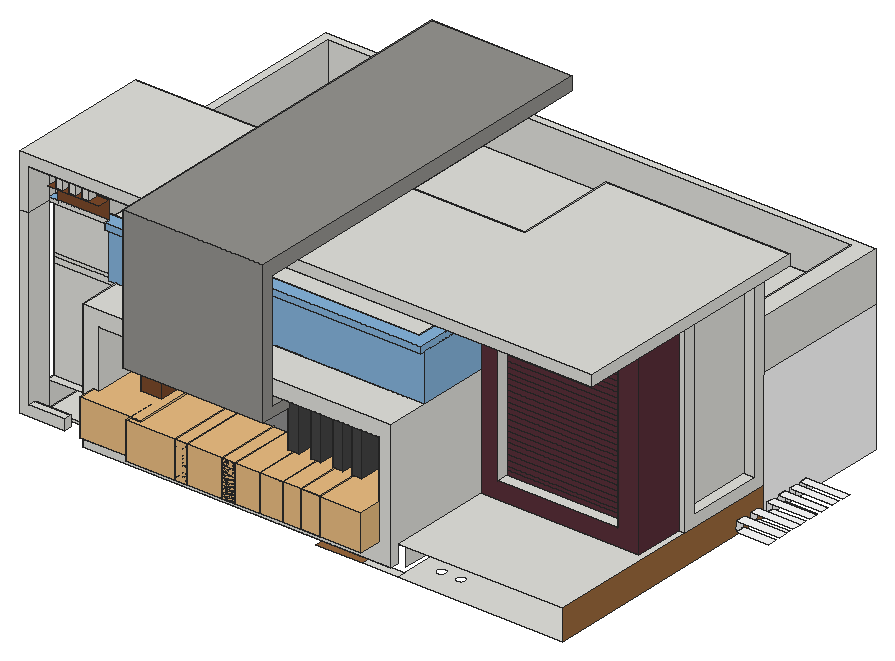
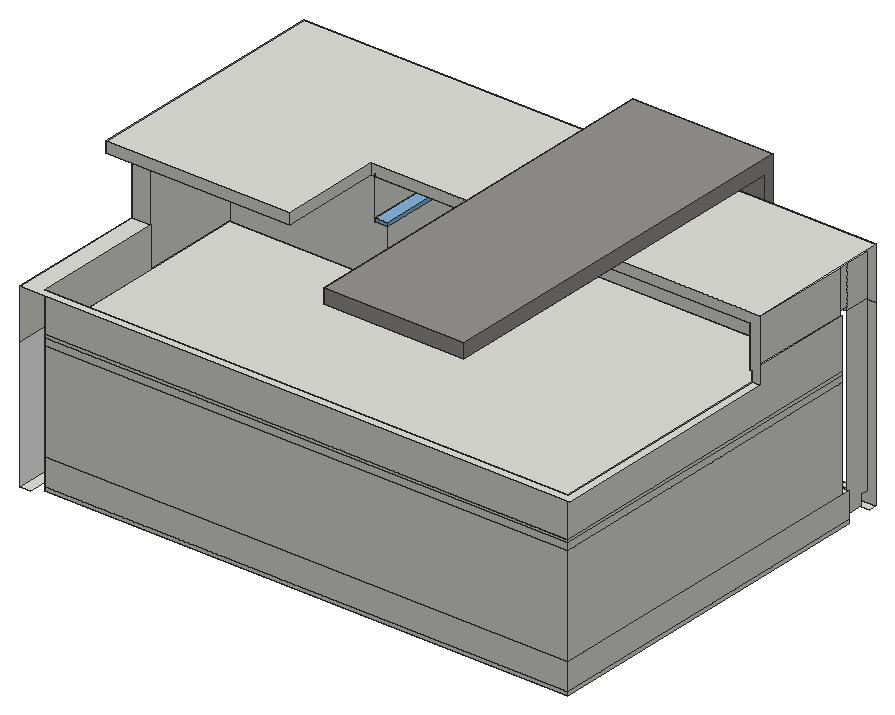
# SketchUp Ruby script. Lengths in inches.
U = 1.inch
M = Sketchup.active_model
def pt(a) = Geom::Point3d.new(a.map { |v| v * U })
def face(e, loops, mat)
  f = e.add_face(loops[0].map { |a| pt(a) })
  loops[1..].each { |l| e.add_face(l.map { |a| pt(a) }).erase! }
  f.material = f.back_material = mat if mat
  f
end
# faces: each face lists its corners as indices into pts; further lists are holes
def faces(e, pts, list, mat = nil) = list.each { |f| face(e, (f[0].is_a?(Array) ? f : [f]).map { |l| l.map { |i| pts[i] } }, mat) }
# xy, xz, yz: faces in a plane at the given z, y or x. An outline is a flat list of corners, or four numbers for a rectangle; further outlines are holes
def ring(l) = l.size == 4 ? [[l[0], l[1]], [l[2], l[1]], [l[2], l[3]], [l[0], l[3]]] : l.each_slice(2).to_a
def flat(e, list, mat, &to3) = list.each { |f| face(e, (f[0].is_a?(Array) ? f : [f]).map { |l| ring(l).map { |u, v| to3.(u, v) } }, mat) }
def xy(e, z, list, mat = nil) = flat(e, list, mat) { |x, y| [x, y, z] }
def xz(e, y, list, mat = nil) = flat(e, list, mat) { |x, z| [x, y, z] }
def yz(e, x, list, mat = nil) = flat(e, list, mat) { |y, z| [x, y, z] }
def lines(e, pts, list) = list.each { |a, b| e.add_line(pt(pts[a]), pt(pts[b])) }
# prism: a flat outline (further loops are holes) pulled along v
def prism(e, loops, v, mat = nil)
  f = face(e, loops, mat); d = Geom::Vector3d.new(v.map { |x| x * U })
  f.pushpull(f.normal.samedirection?(d) ? d.length : -d.length)
end
def box(e, o, s, mat = nil) = prism(e, [[o, [o[0] + s[0], o[1], o[2]], [o[0] + s[0], o[1] + s[1], o[2]], [o[0], o[1] + s[1], o[2]]]], [0, 0, s[2]], mat)
def at(x, y, z, deg = 0) = Geom::Transformation.translation(pt([x, y, z])) * Geom::Transformation.rotation(ORIGIN, Z_AXIS, deg.degrees)
def axes(o, x, y, z) = Geom::Transformation.new([*x, 0, *y, 0, *z, 0, *pt(o).to_a, 1])
def part(name) = M.definitions.add(name)
# library, detail: a bought-in or finely detailed component or shape, given as its bounding box
def library(name, o, s) = part(name).tap { |d| box(d.entities, o, s) }
def detail(e, o, s) = box(e.add_group.entities, o, s)
def put(e, d, t, mat = nil) = e.add_instance(d, t).tap { |i| i.material = mat if mat }
def group(e, t, mat = nil) = e.add_group.tap { |g| g.transformation = t; g.material = mat if mat }.entities
root = M.entities
M.materials.add("[Color I06]").color = [134, 181, 221]
M.materials.add("[Color L16]").color = [89, 47, 58]
M.materials.add("[Color M00]").color = [255, 255, 255]
M.materials.add("[Color M02]").color = [198, 198, 198]
M.materials.add("[Color M03]").color = [186, 170, 170]
M.materials.add("[Color M04]").color = [142, 142, 142]
M.materials.add("[Color M08]").color = [30, 30, 30]
M.materials.add("[Concrete Aggregate Smoke]").color = [154, 150, 148]
M.materials.add("[Granite Dark Gray]").color = [69, 68, 68]
M.materials.add("[Granite Light Gray]").color = [149, 148, 144]
M.materials.add("[Wood Floor Dark]").color = [123, 73, 42]
M.materials.add("[Wood Floor]").color = [155, 105, 61]
c1 = library("SimLab\#1",[-34.39,-41.14,-1.55],[72.52,77.18,43.59])
xy(root,129,[[514.48,231,557.08,241.25],[[557.08,231,754.5,408.375],[582.5,258.46,583.98,258.6,585.375,259.11,586.59,259.96,587.54,261.1,588.16,262.45,588.42,263.91,588.28,265.39,587.77,266.78,586.92,268,585.78,268.95,584.43,269.57,582.97,269.83,581.49,269.69,580.09,269.18,578.88,268.33,577.93,267.1875,577.3,265.84,577.05,264.38,577.18,262.9,577.7,261.51,578.55,260.29,579.69,259.34,581.04,258.72],[605.875,258.46,607.35,258.6,608.75,259.11,609.96,259.96,610.91,261.1,611.54,262.45,611.79,263.91,611.66,265.39,611.15,266.78,610.29,268,609.15,268.95,607.8,269.57,606.34,269.83,604.86,269.69,603.47,269.18,602.25,268.33,601.3,267.1875,600.68,265.84,600.43,264.38,600.56,262.9,601.07,261.51,601.93,260.29,603.07,259.34,604.41,258.72]],[103.75,271.1875,103.75,691.8125,732.0625,691.8125,732.0625,414.375,551.08,414.375,551.08,281.3125,105.9,271.1875],[741.0625,408.375,741.0625,700.8125,754.5625,700.8125,754.5625,533.07,754.5,533.07,754.5,408.375]])
xy(root,129,[[469.85,240.4375,471.69,241.25]],"[Color M08]")
xy(root,129,[[458.61,231,458.61,241.25,469.85,241.25,469.85,240.4375,471.69,240.4375,471.69,241.25,514.48,241.25,514.48,231]],"[Wood Floor]")
xy(root,132.83,[[754.5,490.78,793.62,502.66],[754.5,511.53,793.62,523.41]],"[Color M00]")
xy(root,133,[[103.75,271.1875,105.9,271.1875,551.08,281.3125,551.08,414.375,732.0625,414.375,732.0625,691.8125,103.75,691.8125]])
xy(root,133.42,[[754.5625,536.43,793.62,546.3],[754.5625,554.3,793.62,564.18],[754.5625,570.62,793.62,580.49],[754.5625,586.05,793.62,595.93]],"[Color M00]")
xy(root,138.0625,[[94.75,241.25,148.58,250.25]])
xy(root,143.5625,[[186.49,220.625,198.68,241.25],[201.89,220.625,201.89,231,299.43,231,299.43,241.25,410.97,241.25,410.97,231,557.08,231,557.08,220.625],[186.49,241.25,198.68,271.1875]])
xy(root,143.5625,[[198.68,220.625,201.89,241.25],[201.89,231,299.43,241.25]],"[Color M00]")
xy(root,144.7,[[754.5,490.78,806.8125,502.66],[754.5,511.53,806.8125,523.41],[754.5625,536.43,806.8125,546.3],[754.5625,554.3,806.8125,564.18],[754.5625,570.62,806.8125,580.49],
  [754.5625,586.05,806.8125,595.93]],"[Color M00]")
xy(root,151.07,[[105.9,241.25,148.58,250.25]])
xy(root,165,[[428.74,231,557.08,241.25],[557.08,231,754.5,231,754.5,414.375,747.0625,414.375,747.0625,355.0625,557.08,355.0625],[103.75,271.1875,103.75,281.3125,551.08,281.3125],[557.08,355.0625,747.0625,408.375]])
xy(root,165.8125,[[206.18,220.625,542.15,220.625,542.15,271.1875,501.85,271.1875,501.85,245.25,489.97,245.25,489.97,271.1875,479.54,271.1875,479.54,245.25,466.78,245.25,466.78,271.1875,452.72,271.1875,452.72,245.25,441.16,245.25,441.16,271.1875,426.59,271.1875,426.59,245.25,413.25,245.25,413.25,260.5625,261.48,260.5625,261.48,245.25,236.63,245.25,236.63,271.1875,206.18,271.1875],[236.63,245.25,261.48,271.1875],[413.25,245.25,426.59,271.1875],[441.16,245.25,452.72,271.1875],[466.78,245.25,479.54,271.1875],
  [489.97,245.25,501.85,271.1875],[261.48,260.5625,413.25,271.1875]])
xy(root,178.54,[[741.0625,427.91,754.5,519.53]])
xy(root,184.88,[[576.97,355.0625,721.18,368.875]])
xy(root,207.95,[[261.48,260.5625,413.25,271.1875]],"[Color M04]")
xy(root,266.5625,[[259.0625,190.1875,427.6,228.23]],"[Concrete Aggregate Smoke]")
xy(root,278.87,[[259.0625,202.98,427.6,228.23]],"[Granite Light Gray]")
xy(root,279.1875,[[206.18,220.625,542.15,271.1875]])
xy(root,285,[[236.63,245.25,261.48,271.1875],[413.25,245.25,426.59,271.1875],[441.16,245.25,452.72,271.1875],[466.78,245.25,479.54,271.1875],[489.97,245.25,501.85,271.1875],
  [754.5,533.07,754.5625,700.8125]])
xy(root,293,[[103.75,281.3125,103.75,691.8125,732.0625,691.8125,732.0625,414.375,551.08,414.375,551.08,281.3125]])
xy(root,297,[[186.49,220.625,557.08,271.1875],[103.75,281.3125,542.15,281.3125,542.15,414.375,732.0625,414.375,732.0625,691.8125,103.75,691.8125],[542.15,281.3125,551.08,414.375]])
xy(root,345,[[94.75,415.6875,103.75,415.6875,103.75,691.8125,732.0625,691.8125,732.0625,533.07,754.5,533.07,754.5,700.8125,94.75,700.8125]])
xy(root,354.375,[[178.1875,264.5,557.08,271.1875]],"[Color I06]")
xy(root,357,[[103.75,281.3125,105.9,415.6875]])
xy(root,362,[[178.1875,264.5,557.08,264.5,557.08,414.375,542.15,414.375,542.15,281.3125,105.9,281.3125,105.9,271.1875,178.1875,271.1875]],"[Color I06]")
xy(root,383.8125,[[124.5,257.99,133,268.3],[140.12,257.99,148.62,268.3],[155.87,257.99,164.37,268.3]])
xy(root,383.8125,[[[116.625,255.4375,178.1875,271.1875],[124.5,257.99,133,268.3],[140.12,257.99,148.62,268.3],[155.87,257.99,164.37,268.3]]],"[Wood Floor Dark]")
xy(root,389.37,[[576.97,355.0625,721.18,368.875]])
xy(root,393.92,[[741.0625,427.91,754.5,501.75],[741.0625,501.75,754.5,519.53]])
xy(root,406.125,[[124.5,257.99,133,268.3]])
xy(root,406.875,[[140.12,257.99,148.62,268.3],[155.87,257.99,164.37,268.3]])
xy(root,407.46,[[105.9,241.25,105.9,415.6875,561.12,415.6875,561.12,538.25,732.0625,538.25,732.0625,414.375,754.5,414.375,754.5,533.07,747.0625,533.07,747.0625,538.25,781.08,538.25,781.08,241.25],[732.0625,414.375,754.5,533.07],[732.0625,533.07,747.0625,538.25]])
xy(root,413,[[557.08,355.0625,747.0625,414.375]])
xy(root,419.9375,[[94.75,241.25,259.0625,415.6875],[259.0625,241.25,427.6,415.6875],[427.6,241.25,781.08,241.25,781.08,538.25,561.12,538.25,561.12,415.6875,427.6,415.6875]])
xy(root,419.9375,[[259.0625,415.6875,427.6,654]],"[Concrete Aggregate Smoke]")
xy(root,419.9375,[[259.0625,202.98,427.6,241.25]],"[Granite Light Gray]")
xy(root,437.125,[[259.0625,190.1875,427.6,654]],"[Granite Light Gray]")
xz(root,190.1875,[[259.0625,266.5625,427.6,437.125]],"[Granite Light Gray]")
xz(root,202.98,[[259.0625,278.87,427.6,419.9375]],"[Granite Light Gray]")
xz(root,220.625,[[[186.49,143.5625,557.08,297],[206.18,165.8125,542.15,279.1875]]])
xz(root,228.23,[[259.0625,266.5625,427.6,278.87]])
xz(root,231,[[410.97,143.5625,428.74,165,428.74,143.5625],[428.74,143.5625,557.08,165]])
xz(root,241.25,[[94.75,138.0625,148.58,138.0625,148.58,151.07,105.9,151.07,105.9,357,94.75,357],[94.75,357,105.9,357,105.9,407.46,781.08,407.46,781.08,419.9375,94.75,419.9375]])
xz(root,245.25,[[413.25,165.8125,426.59,285],[441.16,165.8125,452.72,285],[466.78,165.8125,479.54,285],[489.97,165.8125,501.85,285]],"[Granite Dark Gray]")
xz(root,245.25,[[236.63,165.8125,261.48,285]],"[Wood Floor Dark]")
xz(root,250.25,[[105.9,138.0625,148.58,151.07]])
xz(root,257.99,[[124.5,383.8125,133,406.125],[140.12,383.8125,148.62,406.875],[155.87,383.8125,164.37,406.875]])
xz(root,260.5625,[[261.48,165.8125,413.25,192.91],[261.48,192.91,413.25,207.95]],"[Color M04]")
xz(root,264.5,[[178.1875,354.375,557.08,362]],"[Color I06]")
xz(root,268.3,[[124.5,383.8125,133,406.125],[140.12,383.8125,148.62,406.875],[155.87,383.8125,164.37,406.875]])
xz(root,271.1875,[[103.75,129,105.9,133],[103.75,133,105.9,165],[236.63,165.8125,261.48,279.1875],[261.48,165.8125,413.25,207.95],[413.25,165.8125,426.59,279.1875],
  [441.16,165.8125,452.72,279.1875],[466.78,165.8125,479.54,279.1875],[489.97,165.8125,501.85,279.1875],[206.18,279.1875,236.63,285],[236.63,279.1875,261.48,285],
  [261.48,279.1875,413.25,285],[413.25,279.1875,426.59,285],[426.59,279.1875,441.16,285],[441.16,279.1875,452.72,285],[452.72,279.1875,466.78,285],
  [466.78,279.1875,479.54,285],[479.54,279.1875,489.97,285],[489.97,279.1875,501.85,285],[501.85,279.1875,506.47,285],[506.47,279.1875,542.15,285],
  [206.18,285,236.63,297],[236.63,285,261.48,297],[261.48,285,413.25,297],[413.25,285,426.59,297],[426.59,285,441.16,297],
  [441.16,285,452.72,297],[452.72,285,466.78,297],[466.78,285,479.54,297],[479.54,285,489.97,297],[489.97,285,501.85,297],
  [501.85,285,506.47,297],[506.47,285,542.15,297],[105.9,357,116.625,362],[116.625,357,178.1875,362]])
xz(root,271.1875,[[178.1875,297,557.08,354.375]],"[Color I06]")
xz(root,271.1875,[[506.47,165.8125,542.15,279.1875]],"[Color M02]")
xz(root,271.1875,[[206.18,165.8125,236.63,279.1875]],"[Color M03]")
xz(root,271.1875,[[261.48,207.95,413.25,279.1875]],"[Color M04]")
xz(root,271.1875,[[426.59,165.8125,441.16,279.1875],[452.72,165.8125,466.78,279.1875],[479.54,165.8125,489.97,279.1875],[501.85,165.8125,506.47,279.1875]],"[Granite Dark Gray]")
xz(root,271.1875,[[116.625,362,178.1875,383.8125]],"[Wood Floor Dark]")
xz(root,281.3125,[[103.75,165,551.08,285],[103.75,285,551.08,293],[103.75,293,386.36,297],[386.36,293,412.8,297],[412.8,293,551.08,297],
  [103.75,297,542.15,357]])
xz(root,281.3125,[[105.9,357,542.15,362]],"[Color I06]")
xz(root,355.0625,[[[557.08,165,747.0625,413],[576.97,184.88,721.18,389.37]]],"[Color L16]")
xz(root,368.875,[[576.97,184.88,721.18,190.27],[576.97,190.27,721.18,195.33],[576.97,195.33,721.18,201.58],[576.97,201.58,721.18,207.83],[576.97,207.83,721.18,214.08],
  [576.97,214.08,721.18,220.33],[576.97,220.33,721.18,226.58],[576.97,226.58,721.18,232.83],[576.97,232.83,721.18,239.08],[576.97,239.08,721.18,245.33],
  [576.97,245.33,721.18,251.58],[576.97,251.58,721.18,257.83],[576.97,257.83,721.18,264.08],[576.97,264.08,721.18,270.33],[576.97,270.33,721.18,276.58],
  [576.97,276.58,721.18,282.83],[576.97,282.83,721.18,289.08],[576.97,289.08,721.18,295.33],[576.97,295.33,721.18,301.58],[576.97,301.58,721.18,307.83],
  [576.97,307.83,721.18,314.08],[576.97,314.08,721.18,320.33],[576.97,320.33,721.18,326.58],[576.97,326.58,721.18,332.83],[576.97,332.83,721.18,339.08],
  [576.97,339.08,721.18,345.33],[576.97,345.33,721.18,351.58],[576.97,351.58,721.18,357.83],[576.97,357.83,721.18,364.08],[576.97,364.08,721.18,370.33],
  [576.97,370.33,721.18,376.58],[576.97,376.58,721.18,382.83],[576.97,382.83,721.18,389.37]],"[Color L16]")
xz(root,414.375,[[551.08,129,732.0625,133],[551.08,133,732.0625,165],[551.08,165,732.0625,285],[747.0625,165,754.5,407.46],[551.08,285,732.0625,293],
  [551.08,293,732.0625,297],[542.15,297,542.15,357,557.08,357,557.08,413,732.0625,413,732.0625,297],[732.0625,407.46,747.0625,413]])
xz(root,414.375,[[542.15,357,557.08,362]],"[Color I06]")
xz(root,415.6875,[[94.75,345,94.75,419.9375,561.12,419.9375,561.12,407.46,105.9,407.46,105.9,357,103.75,357,103.75,345]])
xz(root,427.91,[[741.0625,178.54,754.5,393.92]])
xz(root,519.53,[[741.0625,178.54,754.5,393.92]])
xz(root,533.07,[[754.5,165,754.5625,285],[732.0625,345,754.5,407.46]])
xz(root,533.07,[[754.5,129,754.5625,165]],"[Wood Floor]")
xz(root,538.25,[[561.12,407.46,781.08,419.9375]])
xz(root,654,[[259.0625,419.9375,427.6,437.125]],"[Concrete Aggregate Smoke]")
xz(root,691.8125,[[103.75,129,732.0625,133],[103.75,133,732.0625,165],[103.75,165,732.0625,285],[103.75,285,732.0625,293],[103.75,293,732.0625,297],
  [103.75,297,732.0625,345]])
yz(root,103.75,[[271.1875,129,691.8125,133],[271.1875,133,691.8125,165],[281.3125,165,691.8125,285],[281.3125,285,691.8125,293],[281.3125,293,691.8125,297],
  [281.3125,297,691.8125,297,691.8125,345,415.6875,345,415.6875,357,281.3125,357]])
yz(root,105.9,[[250.25,138.0625,271.1875,138.0625,271.1875,357,241.25,357,241.25,151.07,250.25,151.07],[241.25,357,271.1875,407.46],[281.3125,357,415.6875,407.46],[271.1875,362,281.3125,407.46]])
yz(root,124.5,[[257.99,383.8125,268.3,406.125]])
yz(root,133,[[257.99,383.8125,268.3,406.125]])
yz(root,140.12,[[257.99,383.8125,268.3,406.875]])
yz(root,148.58,[[241.25,138.0625,250.25,151.07]])
yz(root,148.62,[[257.99,383.8125,268.3,406.875]])
yz(root,155.87,[[257.99,383.8125,268.3,406.875]])
yz(root,164.37,[[257.99,383.8125,268.3,406.875]])
yz(root,178.1875,[[264.5,354.375,271.1875,362]])
yz(root,186.49,[[220.625,143.5625,271.1875,297]])
yz(root,206.18,[[220.625,165.8125,271.1875,279.1875],[241.25,279.1875,271.1875,285]])
yz(root,236.63,[[245.25,165.8125,271.1875,285]],"[Wood Floor Dark]")
yz(root,259.0625,[[190.1875,266.5625,190.1875,437.125,654,437.125,654,419.9375,202.98,419.9375,202.98,278.87,228.23,278.87,228.23,266.5625]],"[Granite Light Gray]")
yz(root,261.48,[[260.5625,165.8125,271.1875,207.95]])
yz(root,261.48,[[245.25,165.8125,260.5625,165.8125,260.5625,207.95,271.1875,207.95,271.1875,285,245.25,285]],"[Wood Floor Dark]")
yz(root,413.25,[[260.5625,165.8125,271.1875,207.95]])
yz(root,413.25,[[245.25,165.8125,245.25,285,271.1875,285,271.1875,207.95,260.5625,207.95,260.5625,165.8125]],"[Granite Dark Gray]")
yz(root,426.59,[[245.25,165.8125,271.1875,285]],"[Granite Dark Gray]")
yz(root,427.6,[[190.1875,266.5625,228.23,266.5625,228.23,278.87,202.98,278.87,202.98,419.9375,654,419.9375,654,437.125,190.1875,437.125]],"[Granite Light Gray]")
yz(root,441.16,[[245.25,165.8125,271.1875,285]],"[Granite Dark Gray]")
yz(root,452.72,[[245.25,165.8125,271.1875,285]],"[Granite Dark Gray]")
yz(root,466.78,[[245.25,165.8125,271.1875,285]],"[Granite Dark Gray]")
yz(root,479.54,[[245.25,165.8125,271.1875,285]],"[Granite Dark Gray]")
yz(root,489.97,[[245.25,165.8125,271.1875,285]],"[Granite Dark Gray]")
yz(root,501.85,[[245.25,165.8125,271.1875,285]],"[Granite Dark Gray]")
yz(root,542.15,[[220.625,165.8125,271.1875,279.1875],[241.25,279.1875,271.1875,285],[281.3125,297,414.375,357]])
yz(root,542.15,[[281.3125,357,414.375,362]],"[Color I06]")
yz(root,551.08,[[250.25,129,281.3125,165],[281.3125,129,414.375,133],[281.3125,133,414.375,165],[281.3125,165,414.375,285],[281.3125,285,414.375,293],
  [281.3125,293,414.375,297]])
yz(root,557.08,[[220.625,143.5625,231,143.5625,231,165,355.0625,165,355.0625,297,220.625,297],[355.0625,357,414.375,362],[355.0625,362,414.375,413]])
yz(root,557.08,[[271.1875,297,355.0625,354.375],[264.5,354.375,355.0625,362]],"[Color I06]")
yz(root,561.12,[[415.6875,407.46,538.25,419.9375]])
yz(root,576.97,[[355.0625,184.88,368.875,389.37]])
yz(root,721.18,[[355.0625,184.88,368.875,389.37]])
yz(root,732.0625,[[414.375,129,691.8125,133],[414.375,133,691.8125,165],[414.375,165,691.8125,285],[414.375,285,691.8125,293],[414.375,293,691.8125,297],
  [414.375,297,533.07,407.46],[533.07,297,691.8125,345]])
yz(root,741.0625,[[427.91,178.54,519.53,393.92]])
yz(root,747.0625,[[355.0625,165,414.375,413]],"[Color L16]")
yz(root,754.5,[[[414.375,165,533.07,407.46],[427.91,178.54,519.53,393.92]],[533.07,285,700.8125,345]])
yz(root,754.5,[[490.78,132.83,502.66,144.7],[511.53,132.83,523.41,144.7]],"[Color M00]")
yz(root,754.5,[[[231,129,533.07,165],[490.78,132.83,502.66,144.7],[511.53,132.83,523.41,144.7]]],"[Wood Floor]")
yz(root,754.5625,[[[533.07,129,700.8125,285],[536.43,133.42,546.3,144.7],[554.3,133.42,564.18,144.7],[570.62,133.42,580.49,144.7],[586.05,133.42,595.93,144.7]],[536.43,133.42,546.3,144.7],[554.3,133.42,564.18,144.7],[570.62,133.42,580.49,144.7],[586.05,133.42,595.93,144.7]],"[Color M00]")
yz(root,781.08,[[241.25,407.46,538.25,419.9375]])
p = [[105.9,271.1875,129],[551.08,281.3125,129],[551.08,281.3125,133],[105.9,271.1875,133],[410.97,231,143.5625],[428.74,231,165],
  [428.74,241.25,165],[410.97,241.25,143.5625],[557.08,408.375,129],[557.08,408.375,165],[206.18,241.25,285],[206.18,220.625,285],
  [542.15,241.25,285],[542.15,220.625,285],[542.15,241.25,297],[557.08,241.25,285],[105.9,271.1875,357],[105.9,281.3125,357],
  [178.1875,271.1875,357],[557.08,271.1875,357]]
faces(root,p,[[0,1,2,3],[4,5,6,7]])
lines(root,p,[[8,9],[10,11],[12,13],[12,14],[12,15],[16,17],[18,19]])
put(root,c1,at(294.67,235.15,167.36))
put(root,c1,at(352.73,235.15,167.36))
put(root,c1,at(409.6,235.15,167.36))
put(root,c1,at(454.54,235.15,167.36))
put(root,c1,at(504.23,235.15,167.36))
put(root,c1,at(234.38,241.39,168.61))
